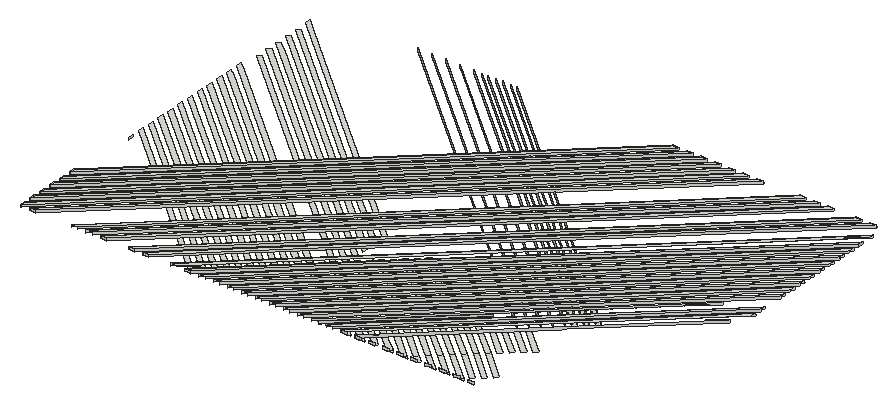
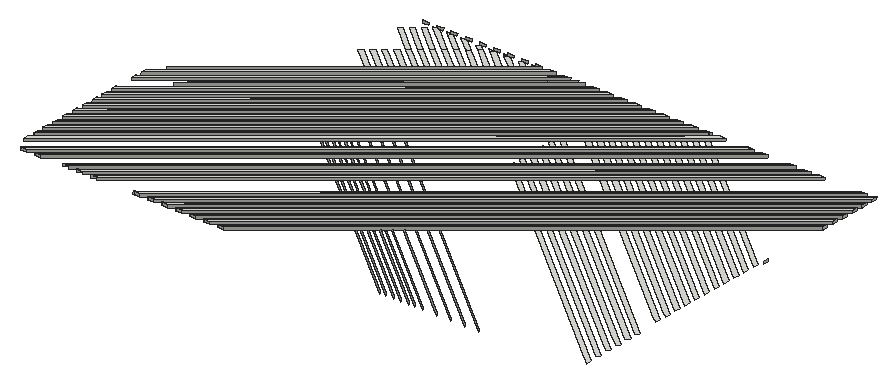
# SketchUp Ruby script. Lengths in inches.
U = 1.inch
M = Sketchup.active_model
def pt(a) = Geom::Point3d.new(a.map { |v| v * U })
def face(e, loops, mat)
  f = e.add_face(loops[0].map { |a| pt(a) })
  loops[1..].each { |l| e.add_face(l.map { |a| pt(a) }).erase! }
  f.material = f.back_material = mat if mat
  f
end
# faces: each face lists its corners as indices into pts; further lists are holes
def faces(e, pts, list, mat = nil) = list.each { |f| face(e, (f[0].is_a?(Array) ? f : [f]).map { |l| l.map { |i| pts[i] } }, mat) }
# xy, xz, yz: faces in a plane at the given z, y or x. An outline is a flat list of corners, or four numbers for a rectangle; further outlines are holes
def ring(l) = l.size == 4 ? [[l[0], l[1]], [l[2], l[1]], [l[2], l[3]], [l[0], l[3]]] : l.each_slice(2).to_a
def flat(e, list, mat, &to3) = list.each { |f| face(e, (f[0].is_a?(Array) ? f : [f]).map { |l| ring(l).map { |u, v| to3.(u, v) } }, mat) }
def xy(e, z, list, mat = nil) = flat(e, list, mat) { |x, y| [x, y, z] }
def xz(e, y, list, mat = nil) = flat(e, list, mat) { |x, z| [x, y, z] }
def yz(e, x, list, mat = nil) = flat(e, list, mat) { |y, z| [x, y, z] }
def lines(e, pts, list) = list.each { |a, b| e.add_line(pt(pts[a]), pt(pts[b])) }
# prism: a flat outline (further loops are holes) pulled along v
def prism(e, loops, v, mat = nil)
  f = face(e, loops, mat); d = Geom::Vector3d.new(v.map { |x| x * U })
  f.pushpull(f.normal.samedirection?(d) ? d.length : -d.length)
end
def box(e, o, s, mat = nil) = prism(e, [[o, [o[0] + s[0], o[1], o[2]], [o[0] + s[0], o[1] + s[1], o[2]], [o[0], o[1] + s[1], o[2]]]], [0, 0, s[2]], mat)
def at(x, y, z, deg = 0) = Geom::Transformation.translation(pt([x, y, z])) * Geom::Transformation.rotation(ORIGIN, Z_AXIS, deg.degrees)
def axes(o, x, y, z) = Geom::Transformation.new([*x, 0, *y, 0, *z, 0, *pt(o).to_a, 1])
def part(name) = M.definitions.add(name)
# library, detail: a bought-in or finely detailed component or shape, given as its bounding box
def library(name, o, s) = part(name).tap { |d| box(d.entities, o, s) }
def detail(e, o, s) = box(e.add_group.entities, o, s)
def put(e, d, t, mat = nil) = e.add_instance(d, t).tap { |i| i.material = mat if mat }
def group(e, t, mat = nil) = e.add_group.tap { |g| g.transformation = t; g.material = mat if mat }.entities
root = M.entities
yz(root,1643.826,[[549.489,108.36,551.842,108.443,551.819,109.47,549.466,109.387]])
yz(root,1888.281,[[640.668,112.65,642.957,112.731,642.934,113.758,640.646,113.677]])
p = [[1780.259,498.812,107.62],[1772.297,491.896,107.375],[1772.297,491.897,107.346],[1773.253,492.728,107.375],[1774.987,494.234,107.428],[1776.304,495.378,107.469],
  [1778.037,496.884,107.522],[1779.392,498.06,107.564],[1780.258,498.813,107.591],[1781.868,491.895,107.346],[1781.868,491.894,107.375],[1781.868,491.871,108.402],
  [1784.577,491.872,108.402],[1784.577,491.894,107.375],[1784.577,491.895,107.346],[1783.781,491.895,107.346],[1782.868,492.688,107.374],[1786.49,491.895,107.346],
  [1784.222,493.865,107.415],[1789.958,491.895,107.346],[1789.004,492.724,107.375],[1788.05,491.895,107.346],[1788.05,491.872,108.402],[1790.679,491.872,108.402],
  [1790.679,491.895,107.375],[1790.679,491.895,107.346],[1796.459,499.2,107.604],[1795.142,498.056,107.564],[1793.408,496.55,107.511],[1792.054,495.373,107.469],
  [1790.321,493.868,107.415],[1884.163,575.372,111.362],[1884.163,575.394,110.335],[1842.51,539.208,109.023],[1841.155,538.031,108.981],[1839.423,536.526,108.928],
  [1838.106,535.382,108.887],[1836.372,533.876,108.834],[1835.018,532.699,108.792],[1833.285,531.194,108.739],[1831.968,530.049,108.698],[1830.234,528.543,108.645],
  [1828.88,527.367,108.603],[1827.147,525.861,108.55],[1825.83,524.717,108.509],[1824.097,523.211,108.456],[1822.742,522.034,108.414],[1821.01,520.529,108.361],
  [1819.693,519.385,108.32],[1817.959,517.879,108.267],[1816.605,516.702,108.225],[1814.872,515.197,108.172],[1813.555,514.053,108.131],[1811.821,512.546,108.078],
  [1810.467,511.37,108.036],[1808.734,509.865,107.983],[1807.417,508.72,107.942],[1805.684,507.214,107.889],[1804.329,506.038,107.847],[1802.597,504.532,107.794],
  [1801.279,503.388,107.753],[1799.546,501.882,107.7],[1798.191,500.705,107.658],[1792.592,491.895,107.346],[1796.058,491.896,107.346],[1797.412,493.072,107.387],
  [1794.144,491.895,107.375],[1794.144,491.872,108.402],[1796.853,491.872,108.402],[1796.853,491.895,107.375],[1796.853,491.896,107.346],[1794.144,491.895,107.346],
  [1797.773,498.058,107.564],[1802.234,491.896,107.346],[1803.552,493.04,107.386],[1807.235,495.204,107.463],[1808.334,491.896,107.346],[1809.154,491.896,107.346],
  [1810.098,492.717,107.375],[1802.955,491.873,108.402],[1802.955,491.895,107.375],[1802.955,491.896,107.346],[1800.321,491.896,107.346],[1800.321,491.895,107.375],
  [1800.321,491.873,108.402],[1803.912,492.727,107.375],[1804.869,491.896,107.346],[1806.421,491.873,108.402],[1809.13,491.873,108.402],[1809.154,491.873,108.402],
  [1806.421,491.896,107.346],[1811.044,491.896,107.346],[1815.828,493.041,107.386],[1813.149,495.368,107.469],[1811.832,494.224,107.428],[1814.511,491.897,107.346],
  [1812.597,491.873,108.402],[1815.232,491.873,108.402],[1815.232,491.896,107.375],[1815.232,491.897,107.346],[1812.597,491.897,107.346],[1812.597,491.896,107.375],
  [1821.407,491.897,107.346],[1823.32,491.897,107.346],[1816.235,498.05,107.564],[1814.881,496.873,107.522],[1820.611,491.897,107.346],[1820.635,491.897,107.346],
  [1828.105,493.042,107.386],[1819.286,500.701,107.658],[1817.969,499.557,107.617],[1826.788,491.897,107.346],[1818.698,491.896,107.375],[1818.698,491.874,108.402],
  [1821.407,491.874,108.402],[1821.407,491.896,107.375],[1818.698,491.897,107.346],[1822.372,503.383,107.753],[1821.018,502.206,107.711],[1832.888,491.898,107.346],
  [1833.683,491.898,107.346],[1834.64,492.729,107.375],[1827.509,491.874,108.402],[1827.509,491.897,107.375],[1827.509,491.897,107.346],[1824.874,491.897,107.346],
  [1824.874,491.897,107.375],[1824.874,491.874,108.402],[1829.422,491.898,107.346],[1833.683,491.875,108.402],[1830.974,491.898,107.346],[1830.974,491.897,107.375],
  [1830.974,491.874,108.402],[1835.597,491.898,107.346],[1837.151,491.898,107.346],[1837.151,491.897,107.375],[1837.151,491.875,108.402],[1839.785,491.875,108.402],
  [1839.785,491.898,107.346],[1839.064,491.898,107.346],[1642.998,493.861,107.445],[1643.01,491.583,107.364],[1643.01,491.56,108.391],[1642.998,493.839,108.472],
  [1829.906,653.92,114.147],[1829.906,653.942,113.12],[1827.272,653.942,113.12],[1649.533,491.886,107.375],[1649.533,491.864,108.402],[1646.824,491.863,108.402],
  [1646.824,491.886,107.375],[1833.372,653.942,113.12],[1833.372,653.92,114.147],[1836.081,653.943,113.12],[1836.081,653.92,114.147],[1851.825,653.944,113.12],
  [1665.278,491.887,107.375],[1665.278,491.865,108.402],[1851.825,653.921,114.147],[1854.459,653.921,114.147],[1667.912,491.865,108.402],[1667.912,491.887,107.375],
  [1854.459,653.944,113.12],[1857.925,653.944,113.12],[1671.378,491.887,107.375],[1671.378,491.865,108.402],[1857.925,653.921,114.147],[1860.634,653.922,114.147],
  [1674.087,491.865,108.402],[1674.087,491.888,107.375],[1860.634,653.944,113.12],[1677.554,491.888,107.375],[1680.189,491.888,107.375],[1680.189,491.865,108.402],
  [1677.554,491.865,108.402],[1864.101,653.944,113.12],[1864.101,653.922,114.147],[1866.736,653.922,114.147],[1866.736,653.944,113.12],[1876.378,653.945,113.12],
  [1689.831,491.889,107.375],[1689.831,491.866,108.402],[1876.378,653.922,114.147],[1879.013,653.945,113.12],[1692.466,491.889,107.375],[1692.466,491.866,108.402],
  [1879.013,653.923,114.147],[1885.187,653.946,113.12],[1698.64,491.889,107.375],[1695.931,491.889,107.375],[1882.478,653.945,113.12],[1695.931,491.866,108.402],
  [1882.478,653.923,114.147],[1698.64,491.867,108.402],[1885.187,653.923,114.147],[1888.28,648.322,112.921],[1708.208,491.89,107.375],[1708.208,491.867,108.402],
  [1888.28,648.299,113.948],[1717.019,491.89,107.375],[1716.459,491.89,107.375],[1714.384,491.89,107.375],[1714.384,491.867,108.402],[1717.019,491.868,108.402],
  [1888.281,640.668,112.65],[1715.421,492.791,107.407],[1888.281,642.957,112.731],[1888.281,640.646,113.677],[1888.281,637.658,112.543],[1720.484,491.89,107.375],
  [1720.484,491.868,108.402],[1888.281,637.636,113.57],[1888.281,635.282,113.486],[1723.193,491.868,108.402],[1723.193,491.891,107.375],[1888.281,635.305,112.459],
  [1888.282,632.293,112.353],[1726.661,491.891,107.375],[1726.661,491.868,108.402],[1888.282,632.271,113.38],[1888.282,629.982,113.298],[1729.296,491.868,108.402],
  [1729.296,491.891,107.375],[1888.282,630.005,112.272],[1888.282,626.995,112.165],[1732.761,491.891,107.375],[1732.761,491.869,108.402],[1888.282,626.972,113.192],
  [1888.282,624.619,113.108],[1735.47,491.869,108.402],[1735.47,491.891,107.375],[1888.282,624.642,112.081],[1888.282,621.63,111.975],[1738.9375,491.892,107.375],
  [1738.9375,491.869,108.402],[1888.282,621.607,113.002],[1888.283,619.319,112.92],[1741.572,491.869,108.402],[1741.572,491.892,107.375],[1888.283,619.341,111.894],
  [1888.283,616.331,111.787],[1745.038,491.892,107.375],[1745.038,491.869,108.402],[1888.283,616.309,112.814],[1888.283,613.956,112.73],[1747.747,491.869,108.402],
  [1747.747,491.892,107.375],[1888.283,613.978,111.703],[1888.283,610.966,111.597],[1751.214,491.892,107.375],[1751.214,491.87,108.402],[1888.283,610.944,112.624],
  [1888.283,608.655,112.542],[1753.849,491.87,108.402],[1753.849,491.892,107.375],[1888.283,608.678,111.515],[1888.284,605.668,111.409],[1757.314,491.893,107.375],
  [1757.314,491.87,108.402],[1888.284,605.645,112.436],[1888.284,603.292,112.352],[1760.023,491.87,108.402],[1760.023,491.893,107.375],[1888.284,603.315,111.325],
  [1888.284,600.303,111.219],[1763.491,491.893,107.375],[1763.491,491.87,108.402],[1888.284,600.28,112.245],[1888.284,597.992,112.164],[1766.125,491.871,108.402],
  [1766.125,491.893,107.375],[1888.284,598.014,111.137],[1871.05,580.032,110.5],[1769.591,491.893,107.375],[1769.591,491.871,108.402],[1871.05,580.01,111.527],
  [1874.935,583.385,111.646],[1874.935,583.408,110.62],[1772.3,491.871,108.402],[1780.262,498.787,108.647],[1888.285,589.639,110.84],[1775.767,491.894,107.375],
  [1775.767,491.871,108.402],[1888.285,589.617,111.867],[1778.402,491.894,107.375],[1888.285,587.351,110.759],[1888.285,587.328,111.786],[1778.402,491.871,108.402],
  [1847.252,548.695,109.389],[1888.285,584.318,111.68],[1888.285,584.341,110.653],[1783.117,494.825,107.449],[1781.301,494.049,107.422],[1787.273,496.515,107.509],
  [1785.956,495.371,107.469],[1888.281,642.934,113.758],[1715.421,492.768,108.434],[1716.467,493.677,108.466],[1643.01,493.849,108.472],[1827.272,653.92,114.147],
  [1714.93,495.367,107.469],[1643.826,557.119,109.658],[1643.826,554.831,109.577],[1713.613,494.222,107.428],[1744.302,520.884,108.373],[1745.619,522.028,108.414],
  [1812.161,496.226,107.499],[1837.69,495.38,107.469],[1836.074,496.783,107.519],[1825.423,506.034,107.847],[1824.106,504.889,107.806],[1836.373,494.236,107.428],
  [1645.138,619.979,110.859],[1753.931,525.494,107.509],[1753.931,523.206,107.428],[1643.821,618.834,110.818],[1784.865,498.606,107.583],[1782.442,500.71,107.658],
  [1781.125,499.566,107.617],[1782.862,498.058,107.564],[1785.53,503.392,107.753],[1784.175,502.215,107.711],[1788.048,501.205,107.676],[1718.017,498.048,107.564],
  [1643.825,562.483,109.848],[1643.825,560.13,109.765],[1716.663,496.872,107.522],[1747.351,523.533,108.467],[1748.706,524.71,108.509],[1840.777,498.062,107.564],
  [1828.509,508.716,107.942],[1827.155,507.539,107.9],[1836.336,499.566,107.617],[1839.423,496.885,107.522],[1642.997,496.872,107.552],[1643.009,499.236,107.635],
  [1643.009,499.213,108.662],[1642.997,496.849,108.579],[1643.01,496.86,108.579],[1643.014,496.887,107.552],[1823.804,653.942,113.12],[1823.804,653.919,114.147],
  [1643.014,496.864,108.579],[1643.026,499.25,107.636],[1821.095,653.942,113.12],[1787.263,504.898,107.807],[1788.581,506.042,107.847],[1817.087,530.804,108.755],
  [1790.313,507.547,107.9],[1791.668,508.724,107.942],[1793.401,510.23,107.996],[1794.719,511.374,108.036],[1796.451,512.879,108.089],[1797.806,514.056,108.131],
  [1799.539,515.562,108.185],[1800.857,516.706,108.225],[1802.589,518.211,108.278],[1803.944,519.388,108.32],[1805.677,520.894,108.374],[1806.995,522.038,108.414],
  [1808.727,523.543,108.468],[1810.082,524.72,108.509],[1811.816,526.226,108.5625],[1813.133,527.37,108.603],[1814.866,528.875,108.657],[1816.22,530.052,108.698],
  [1817.087,530.805,108.725],[1817.09,530.779,109.781],[1643.026,499.228,108.663],[1821.095,653.919,114.147],[1721.068,500.699,107.658],[1643.825,567.783,110.036],
  [1643.825,565.494,109.955],[1719.751,499.555,107.617],[1750.439,526.216,108.562],[1751.757,527.36,108.603],[1843.828,500.712,107.658],[1831.56,511.367,108.036],
  [1830.243,510.222,107.995],[1842.511,499.568,107.618],[1645.175,625.309,111.048],[1753.931,530.858,107.699],[1753.931,528.505,107.616],[1643.82,624.133,111.006],
  [1817.63,653.919,114.147],[1643.041,502.251,108.77],[1643.025,502.237,108.77],[1643.025,502.26,107.743],[1643.041,502.274,107.743],[1817.63,653.942,113.12],
  [1643.037,504.559,107.824],[1643.037,504.537,108.851],[1724.155,503.381,107.753],[1643.824,573.146,110.226],[1643.825,570.793,110.143],[1722.801,502.204,107.711],
  [1753.489,528.866,108.656],[1754.844,530.042,108.698],[1815.742,506.788,107.874],[1643.053,504.573,107.825],[1814.995,653.941,113.12],[1827.1875,531.212,107.712],
  [1778.488,573.506,109.211],[1685.854,653.957,112.063],[1685.854,653.934,113.09],[1791.67,562.036,109.832],[1822.358,535.384,108.887],[1827.1875,531.189,108.739],
  [1643.053,504.55,108.852],[1814.995,653.919,114.147],[1727.206,506.031,107.847],[1643.824,578.446,110.414],[1643.824,576.158,110.333],[1725.889,504.887,107.806],
  [1756.577,531.548,108.751],[1757.894,532.693,108.792],[1801.281,508.684,107.941],[1802.636,509.861,107.982],[1830.238,533.862,107.806],[1784.59,573.507,109.211],
  [1691.956,653.957,112.063],[1691.956,653.935,113.09],[1794.72,564.686,109.926],[1825.409,538.034,108.981],[1830.238,533.84,108.833],[1648.227,627.959,111.142],
  [1753.93,536.158,107.887],[1753.93,533.869,107.806],[1643.82,629.498,111.196],[1645.137,630.642,111.237],[1730.293,508.713,107.942],[1643.824,583.81,110.604],
  [1643.824,581.456,110.521],[1728.938,507.536,107.9],[1759.627,534.198,108.845],[1760.981,535.374,108.887],[1643.052,507.584,107.931],[1643.064,509.948,108.015],
  [1643.053,507.585,107.931],[1643.081,509.962,108.016],[1643.068,507.598,107.932],[1811.527,653.941,113.12],[1808.818,653.941,113.12],[1643.053,507.5625,108.958],
  [1643.064,509.925,109.042],[1643.068,507.576,108.959],[1811.527,653.919,114.147],[1833.325,536.544,107.901],[1790.765,573.507,109.211],[1698.131,653.958,112.063],
  [1698.131,653.935,113.09],[1797.807,567.368,110.021],[1828.496,540.716,109.076],[1833.325,536.522,108.928],[1643.065,509.926,109.042],[1643.081,509.939,109.043],
  [1808.818,653.918,114.147],[1733.344,511.363,108.036],[1643.823,589.11,110.792],[1643.823,586.821,110.711],[1732.026,510.219,107.995],[1762.715,536.881,108.94],
  [1764.032,538.025,108.981],[1649.324,632.369,111.298],[1753.93,541.521,108.077],[1753.93,539.168,107.994],[1643.82,634.796,111.384],[1645.174,635.973,111.426],
  [1707.751,650.903,111.955],[1704.233,653.958,112.063],[1704.233,653.935,113.09],[1800.858,570.019,110.115],[1831.547,543.366,109.17],[1836.376,539.172,109.022],
  [1836.376,539.194,107.995],[1796.867,573.507,109.211],[1736.43,514.045,108.131],[1643.823,594.473,110.982],[1643.823,592.12,110.899],[1735.076,512.869,108.089],
  [1765.765,539.53,109.034],[1767.119,540.707,109.076],[1833.292,512.872,108.089],[1834.646,514.049,108.131],[1643.08,512.972,108.122],[1643.092,515.271,108.204],
  [1643.081,512.973,108.122],[1643.081,512.95,109.149],[1643.092,515.248,109.231],[1643.108,515.284,108.204],[1643.096,512.986,108.123],[1643.096,512.963,109.15],
  [1805.353,653.941,113.12],[1805.353,653.918,114.147],[1802.718,653.941,113.12],[1803.042,573.508,109.211],[1710.407,653.958,112.063],[1710.407,653.936,113.09],
  [1803.945,572.7,110.21],[1834.634,546.048,109.265],[1839.463,541.854,109.117],[1839.463,541.876,108.09],[1806.509,573.508,109.211],[1841.197,543.382,108.143],
  [1841.197,543.36,109.17],[1836.368,547.554,109.319],[1805.679,574.206,110.264],[1713.875,653.936,113.09],[1713.875,653.959,112.063],[1809.144,573.508,109.211],
  [1842.514,544.527,108.184],[1643.093,515.249,109.231],[1643.108,515.262,109.231],[1802.718,653.918,114.147],[1643.823,597.485,111.089],[1738.164,515.551,108.184],
  [1739.481,516.696,108.225],[1643.822,599.773,111.17],[1768.852,542.213,109.129],[1770.17,543.357,109.17],[1836.38,515.555,108.184],[1837.697,516.7,108.225],
  [1645.136,641.306,111.615],[1753.929,546.821,108.265],[1753.93,544.533,108.184],[1643.819,640.161,111.574],[1716.509,653.959,112.063],[1716.509,653.936,113.09],
  [1806.996,575.351,110.304],[1837.685,548.698,109.359],[1842.514,544.504,109.211],[1812.609,573.508,109.211],[1844.247,546.032,108.237],[1844.247,546.009,109.264],
  [1839.418,550.203,109.413],[1808.728,576.856,110.358],[1719.975,653.936,113.09],[1719.975,653.959,112.063],[1815.318,573.508,109.211],[1845.601,547.208,108.279],
  [1643.822,602.783,111.277],[1741.214,518.201,108.278],[1742.568,519.378,108.32],[1645.469,603.706,111.31],[1645.177,603.96,111.319],[1643.822,605.136,111.36],
  [1773.257,546.039,109.265],[1771.902,544.862,109.223],[1800.43,520.087,108.345],[1839.429,518.205,108.278],[1840.783,519.382,108.32],[1643.107,518.296,108.311],
  [1643.119,520.66,108.395],[1643.109,518.298,108.311],[1643.135,520.674,108.395],[1643.123,518.31,108.312],[1643.123,518.287,109.339],[1643.109,518.275,109.338],
  [1799.251,653.94,113.12],[1799.251,653.918,114.147],[1643.119,520.637,109.422],[1796.542,653.94,113.12],[1722.684,653.959,112.063],[1722.684,653.937,113.09],
  [1810.083,578.033,110.399],[1840.772,551.379,109.454],[1845.601,547.186,109.306],[1818.786,573.509,109.211],[1847.335,548.714,108.332],[1847.335,548.692,109.359],
  [1842.506,552.885,109.508],[1811.816,579.539,110.453],[1726.151,653.937,113.09],[1726.151,653.959,112.063],[1821.42,573.509,109.211],[1848.652,549.859,108.373],
  [1710.917,491.867,108.402],[1888.281,645.946,113.864],[1710.929,491.867,108.402],[1872.478,578.897,111.487],[1772.293,491.871,108.402],[1888.286,581.965,111.596],
  [1788.044,491.872,108.402],[1643.121,520.639,109.422],[1643.135,520.651,109.422],[1796.542,653.918,114.147],[1643.822,608.148,111.467],[1645.816,608.705,111.487],
  [1645.139,609.293,111.508],[1643.822,610.437,111.548],[1774.99,547.545,109.318],[1776.307,548.689,109.359],[1842.517,520.888,108.373],[1843.834,522.033,108.414],
  [1753.929,549.831,108.372],[1643.819,645.46,111.762],[1643.819,647.813,111.845],[1645.173,646.636,111.804],[1649.496,642.882,111.671],[1753.929,552.184,108.455],
  [1728.786,653.959,112.063],[1728.786,653.937,113.09],[1813.133,580.683,110.493],[1843.823,554.03,109.548],[1848.652,549.836,109.4],[1825.414,495.378,107.499],
  [1827.148,493.872,107.445]]
faces(root,p,[[0,1,2,3,4,5,6,7,8],[9,10,11,12,13,14,15],[16,15,14,17,18],[19,20,21],[21,22,23,24,25,19],[26,27,28,29,30,20,21,22,31,32,33,34,35,36,37,38,39,40,41,42,43,44,45,46,47,48,49,50,51,52,53,54,55,56,57,58,59,60,61,62],[25,63,30,20,19],[28,29,64,65],
  [66,67,68,69,70,64,71],[72,26,27,73,74],[75,61,62,76,77,78],[79,80,81,73,82,83,84],[81,85,74,73],[85,81,86],[87,88,89,77,76,90],[78,77,91],
  [92,93,94,95],[96,97,98,99,95,100,101],[102,103,104,105,106,107],[108,109,110,111],[112,113,114,115,102,107,106,116],[117,118,119,120,121],[122,123,124,111,125,126,127],[124,128,108,111],
  [129,120,119,130,131,132],[120,121,133],[134,135,136,137,138,139],[140,141,142,143],[144,142,141,145],[145,141,140,146],[147,148,149,150],[151,150,149,152],
  [153,147,150,151],[154,148,147,153],[155,156,157,158],[159,160,161,162],[163,164,165,166],[167,168,169,170],[171,172,173,174],[175,171,174,176],
  [177,173,172,178],[179,180,181,182],[183,184,180,179],[180,181,185,184],[186,185,184,183],[187,188,189,190],[190,189,191,192],[188,193,191,189],
  [194,193,188,187],[195,196,197,198],[199,200,201,202,203],[204,199,200,205,206],[207,203,199,204],[208,209,210,211],[212,213,214,215],[216,217,218,219],
  [220,221,222,223],[224,225,226,227],[228,229,230,231],[232,233,234,235],[236,237,238,239],[240,241,242,243],[244,245,246,247],[248,249,250,251],
  [252,253,254,255],[256,257,258,259],[260,261,262,263],[264,265,266,267],[268,269,270,271],[272,273,274,275,276,277],[278,1,0,279],[280,281,282,283],
  [284,285,286,287],[288,10,11,289,290],[291,7,6,292,16,18],[30,293,294,20],[295,206,205,296,297],[146,140,298,299],[300,301,302,303],[304,4,5,305],
  [306,59,60,94,93],[307,308,309,310,311],[312,313,314,315],[316,317,318,319,294,293],[320,321,29,28,322],[323,324,325,326],[327,6,7,328],[104,57,58,105],
  [329,330,331,332,333],[334,335,336,337],[338,337,334,339,340,341,342],[340,339,343,344],[335,343,339,334],[345,27,26,346],[347,0,8,318,317,321,320,345,346,348,349,350,351,352,353,354,355,356,357,358,359,360,361,362,363,364,365,366],[279,0,347,367],
  [343,335,336,368,369,344],[370,371,372,373],[374,318,317,375],[109,55,56,110],[376,377,378,379],[380,381,382,383],[348,62,61,349],[384,385,386,387,388,389],
  [390,391,386,387],[392,393,394,395],[396,321,320,397],[117,53,54,398,118],[390,399,388,387],[389,388,399,400],[401,402,403,404,405,406,407],[350,60,59,351],
  [399,390,391,408,409,400],[410,411,412,413],[414,345,346,415],[309,51,52,310],[416,58,57,417],[418,419,420,421,422,423,424],[425,426,427,428,429],[430,431,432,433],
  [434,348,349,435],[330,49,50,331],[436,437,438],[437,439,440,438],[441,440,439,442],[443,438,437,444],[445,443,438,440,441,446],[417,353,352,416],
  [354,56,55,355],[447,448,449,450,451,452,453],[439,437,444,454,455,456,442],[457,458,459,460],[461,350,351,462],[377,47,48,378],[356,54,53,357],[463,464,465,466,467],
  [468,469,470,471,472,473,474,475],[476,477,478,479],[480,352,353,481],[482,483,45,46],[484,485,486],[485,486,487,488],[485,489,490,486],[491,487,486,490,492,493],
  [492,490,489,494],[358,52,51,359],[495,496,497,498,499,500,501],[502,503,504,505,506,507,508],[503,502,509,510],[489,485,488,511,512,513,494],[514,515,516,517],[518,354,355,519],
  [520,521,43,44],[360,50,49,361],[522,523,524,525],[509,526,527,528,529,530,510],[531,532,533,534,535,536,537],[532,531,538,539],[540,541,542,543,544,545],[356,357,546,547,548],
  [549,550,41,42],[551,552,553],[552,554,555,553],[556,557,553,555,558,559],[557,560,552,553],[558,555,554,561],[362,48,47,363],[538,562,563,564,565,566,539],
  [567,568,569,570,571,572,573],[568,567,574,575],[299,298,142,144],[152,149,148,154],[158,157,160,159],[166,165,168,167],[176,174,173,177],[182,181,185,186],
  [192,191,193,194],[198,197,576,577],[578,577,576],[297,296,202,203,207,295],[211,210,213,212],[219,218,221,220],[227,226,229,228],[235,234,237,236],
  [243,242,245,244],[251,250,253,252],[259,258,261,260],[267,266,269,268],[278,279,579,580],[283,282,287,286],[289,11,12,581],[582,22,31],
  [554,552,560,583,584,585,561],[586,304,305,587,588,589],[590,358,359,591],[592,593,39,40],[594,595,596,597,598,599],[574,600,601,602,603,604,575],[337,338,336],[369,368,342,341],
  [338,342,368,336],[408,391,386,385,384,409],[455,454,443,445,446,456],[454,444,443],[512,511,487,491,493,513],[511,488,487],[584,583,557,556,559,585],[583,560,557],
  [585,559,558,561],[513,493,492,494],[456,446,441,442],[409,384,389,400],[369,341,340,344],[299,144,145,146],[152,154,153,151],[182,186,183,179],
  [192,194,187,190]])
lines(root,p,[[594,523],[465,426],[427,381],[382,313],[524,464],[605,606]])
